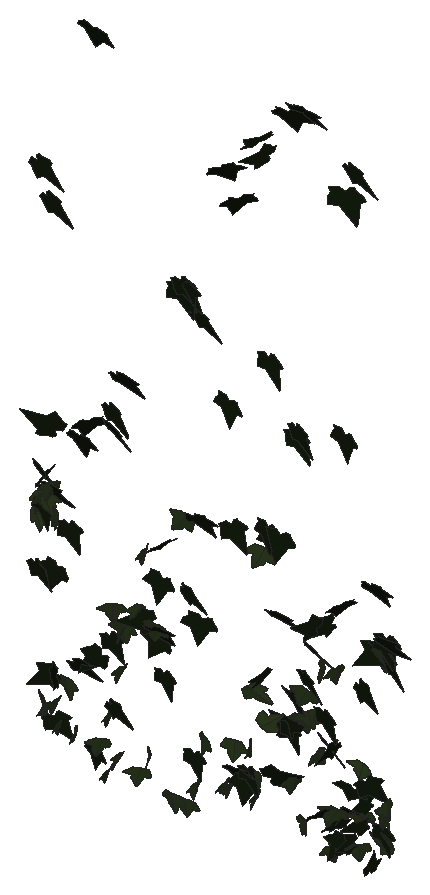
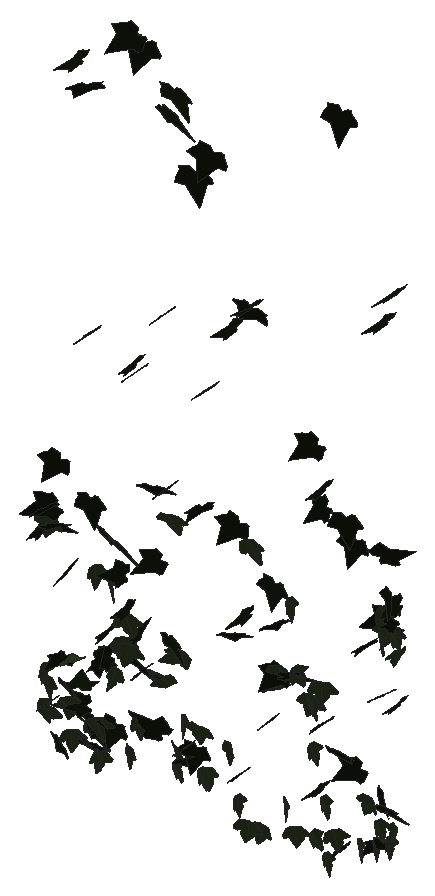
# SketchUp Ruby script. Lengths in inches.
U = 1.inch
M = Sketchup.active_model
def pt(a) = Geom::Point3d.new(a.map { |v| v * U })
def face(e, loops, mat)
  f = e.add_face(loops[0].map { |a| pt(a) })
  loops[1..].each { |l| e.add_face(l.map { |a| pt(a) }).erase! }
  f.material = f.back_material = mat if mat
  f
end
# faces: each face lists its corners as indices into pts; further lists are holes
def faces(e, pts, list, mat = nil) = list.each { |f| face(e, (f[0].is_a?(Array) ? f : [f]).map { |l| l.map { |i| pts[i] } }, mat) }
# xy, xz, yz: faces in a plane at the given z, y or x. An outline is a flat list of corners, or four numbers for a rectangle; further outlines are holes
def ring(l) = l.size == 4 ? [[l[0], l[1]], [l[2], l[1]], [l[2], l[3]], [l[0], l[3]]] : l.each_slice(2).to_a
def flat(e, list, mat, &to3) = list.each { |f| face(e, (f[0].is_a?(Array) ? f : [f]).map { |l| ring(l).map { |u, v| to3.(u, v) } }, mat) }
def xy(e, z, list, mat = nil) = flat(e, list, mat) { |x, y| [x, y, z] }
def xz(e, y, list, mat = nil) = flat(e, list, mat) { |x, z| [x, y, z] }
def yz(e, x, list, mat = nil) = flat(e, list, mat) { |y, z| [x, y, z] }
def lines(e, pts, list) = list.each { |a, b| e.add_line(pt(pts[a]), pt(pts[b])) }
# prism: a flat outline (further loops are holes) pulled along v
def prism(e, loops, v, mat = nil)
  f = face(e, loops, mat); d = Geom::Vector3d.new(v.map { |x| x * U })
  f.pushpull(f.normal.samedirection?(d) ? d.length : -d.length)
end
def box(e, o, s, mat = nil) = prism(e, [[o, [o[0] + s[0], o[1], o[2]], [o[0] + s[0], o[1] + s[1], o[2]], [o[0], o[1] + s[1], o[2]]]], [0, 0, s[2]], mat)
def at(x, y, z, deg = 0) = Geom::Transformation.translation(pt([x, y, z])) * Geom::Transformation.rotation(ORIGIN, Z_AXIS, deg.degrees)
def axes(o, x, y, z) = Geom::Transformation.new([*x, 0, *y, 0, *z, 0, *pt(o).to_a, 1])
def part(name) = M.definitions.add(name)
# library, detail: a bought-in or finely detailed component or shape, given as its bounding box
def library(name, o, s) = part(name).tap { |d| box(d.entities, o, s) }
def detail(e, o, s) = box(e.add_group.entities, o, s)
def put(e, d, t, mat = nil) = e.add_instance(d, t).tap { |i| i.material = mat if mat }
def group(e, t, mat = nil) = e.add_group.tap { |g| g.transformation = t; g.material = mat if mat }.entities
root = M.entities
M.materials.add("1026 AP 7946 SUNNY SIDE UP").color = [254, 231, 186]
M.materials.add("efeu1").color = [18, 25, 13]
M.materials.add("efeu2").color = [43, 57, 29]
c1 = part("ivyleaf_10")
p = [[0,0.5,-0.03],[-0.0625,2.02,-0.43],[-0.19,2.01,-0.46],[-0.54,1.05,-0.29],[-0.52,0.625,-0.18],[-0.83,0.76,-0.28],
  [-1.16,0.64,-0.33],[-1.15,0.33,-0.24],[-0.77,-0.39,0.02],[-0.3,-0.51,0.16],[0.04,-0.48,0.23],[-0.02,2.01,-0.4375],
  [-0.06,2.01,-0.43],[0.04,-0.49,0.23],[0.67,-0.49,0.14],[1.38,0.36,-0.2],[1.375,0.51,-0.24],[0.81,0.65,-0.19],
  [0.62,0.59,-0.15],[0.6,1.09,-0.28],[0.5,1.23,-0.31]]
faces(c1.entities,p,[[0,1,2,3,4,5,6,7,8,9,10],[11,12,0,13,14,15,16,17,18,19,20]],"efeu2")
c2 = part("ivyleaf_9")
p = [[1.54,2.16,1.25],[1.36,2.04,1.19],[-0.21,0.99,0.68],[-0.71,1.11,0.82],[-0.85,0.86,0.67],[-0.8,0.17,0.21],
  [-0.9,-0.01,0.1],[-0.67,-0.16,-0.02],[-0.08,-0.08,-0.05],[-0.03,-0.6,-0.4],[0.65,-0.88,-0.66],[0.83,-0.6,-0.49],
  [1.29,-0.42,-0.43],[1.8125,-0.07,-0.26],[1.21,0.44,0.15]]
faces(c2.entities,p,[[0,1,2,3,4,5,6,7,8,9,10,11,12,13,14]],"efeu1")
put(root,c1,axes([121.33,212.79,302.52],[0.10637,0.39079,-0.00968],[0.02001,-0.01398,-0.40837],[-0.61442,0.0672,-0.01498]),"1026 AP 7946 SUNNY SIDE UP")
put(root,c1,axes([121.55,212.8125,303.32],[0.06673,-0.37905,0.11263],[0.06236,-0.10747,-0.39263],[0.61813,0.05177,0.02745]),"1026 AP 7946 SUNNY SIDE UP")
put(root,c2,axes([121.34,212.72,299.95],[0.26024,-0.34424,-0.06742],[-0.02451,0.06291,-0.39289],[0.54987,0.16572,0.01439]),"1026 AP 7946 SUNNY SIDE UP")
put(root,c2,axes([121.39,212.77,304.82],[0.50632,-0.2219,-0.1012],[-0.11938,0.0607,-0.40245],[0.36159,0.33077,0.00883]),"1026 AP 7946 SUNNY SIDE UP")
put(root,c2,axes([122.21,212.83,306.92],[-0.05078,0.03558,0.41858],[-0.63945,0.02571,-0.03548],[-0.04487,-0.40658,0.03198]),"1026 AP 7946 SUNNY SIDE UP")
put(root,c1,axes([121.73,212.61,293.58],[-0.33327,0.29751,-0.06698],[0.04015,-0.06364,-0.37633],[-0.47774,-0.21289,0.0151]),"1026 AP 7946 SUNNY SIDE UP")
put(root,c2,axes([122.14,212.97,294.69],[-0.5677,0.0109,0.06133],[-0.0946,-0.02922,-0.37094],[-0.00938,-0.36474,0.0294]),"1026 AP 7946 SUNNY SIDE UP")
put(root,c1,axes([121.87,212.75,293.03],[0.00756,-0.36104,-0.03336],[0.0595,0.03067,-0.36972],[0.56658,0.0016,0.03927]),"1026 AP 7946 SUNNY SIDE UP")
put(root,c2,axes([121.65,212.84,303.01],[0.0399,-0.38612,0.09331],[0.00278,-0.09285,-0.39916],[0.62441,0.02508,-0.00419]),"1026 AP 7946 SUNNY SIDE UP")
put(root,c2,axes([121.55,212.65,319.99],[0.37125,-0.34932,-0.17132],[-0.0289,0.18222,-0.42522],[0.60632,0.22258,0.08463]),"1026 AP 7946 SUNNY SIDE UP")
put(root,c1,axes([121.85,212.78,303.5],[-0.54402,-0.18187,-0.0849],[0.20368,-0.0814,-0.38039],[0.23805,-0.34598,0.13143]),"1026 AP 7946 SUNNY SIDE UP")
put(root,c2,axes([122.06,212.32,304.62],[0.02868,0.31316,0.28228],[0.05693,0.27025,-0.32119],[-0.64997,0.03749,-0.01568]),"1026 AP 7946 SUNNY SIDE UP")
put(root,c1,axes([122.23,212.74,304.17],[-0.16107,-0.37373,0.10448],[0.00803,-0.10838,-0.39845],[0.60974,-0.0973,0.03285]),"1026 AP 7946 SUNNY SIDE UP")
put(root,c2,axes([121.84,212.72,303.97],[0.60813,-0.03029,0.10695],[0.15812,-0.04285,-0.39839],[0.06327,0.39819,-0.03237]),"1026 AP 7946 SUNNY SIDE UP")
put(root,c2,axes([122.63,212.46,294.99],[-0.04508,0.04129,-0.39829],[-0.58566,0.10915,0.04108],[0.17673,0.37224,0.03452]),"1026 AP 7946 SUNNY SIDE UP")
put(root,c2,axes([122.33,212.91,300.04],[-0.1812,-0.33573,0.14976],[-0.00027,-0.15433,-0.36347],[0.57646,-0.1056,0.0469]),"1026 AP 7946 SUNNY SIDE UP")
put(root,c1,axes([122.5,212.68,293.6],[0.01008,-0.37059,0.02268],[-0.00408,-0.02417,-0.38197],[0.58394,0.00623,-0.00306]),"1026 AP 7946 SUNNY SIDE UP")
put(root,c2,axes([122.11,212.67,318.38],[0.3947,-0.35863,-0.10135],[-0.00699,0.11337,-0.44606],[0.58386,0.2438,0.06317]),"1026 AP 7946 SUNNY SIDE UP")
put(root,c1,axes([122.54,212.55,302.875],[0.33528,-0.29784,-0.17526],[-0.06636,0.17406,-0.3711],[0.53392,0.20867,0.06394]),"1026 AP 7946 SUNNY SIDE UP")
put(root,c2,axes([122.45,212.66,292.78],[0.0045,-0.24534,-0.2768],[0.08535,0.26459,-0.24804],[0.56408,-0.03807,0.03974]),"1026 AP 7946 SUNNY SIDE UP")
put(root,c1,axes([122.73,212.61,292.625],[0.07917,-0.35089,-0.09058],[0.01544,0.08806,-0.364],[0.56784,0.04653,0.02252]),"1026 AP 7946 SUNNY SIDE UP")
put(root,c1,axes([122.96,212.82,294.67],[-0.51029,0.1557,-0.08413],[0.06055,-0.10614,-0.36284],[-0.2704,-0.3176,0.07751]),"1026 AP 7946 SUNNY SIDE UP")
put(root,c2,axes([123.02,212.92,302.34],[0.06958,-0.38131,-0.08499],[-0.00634,0.08039,-0.39495],[0.6127,0.04413,0.00557]),"1026 AP 7946 SUNNY SIDE UP")
put(root,c1,axes([123.51,212.72,292.36],[0.11564,-0.32495,-0.14498],[-0.04094,0.13649,-0.3424],[0.55415,0.07789,0.00496]),"1026 AP 7946 SUNNY SIDE UP")
put(root,c2,axes([123.71,212.74,307.09],[0.55846,0.04574,-0.20647],[-0.30488,-0.05996,-0.36794],[-0.10861,0.40351,-0.02883]),"1026 AP 7946 SUNNY SIDE UP")
put(root,c2,axes([123.67,212.6,295.91],[0.58034,0.04904,0.07753],[0.12618,-0.03962,-0.38048],[-0.06264,0.37453,-0.04815]),"1026 AP 7946 SUNNY SIDE UP")
put(root,c2,axes([124.23,212.75,308.01],[0.17855,0.37794,-0.12977],[-0.01863,-0.12995,-0.4065],[-0.62721,0.11145,-0.02487]),"1026 AP 7946 SUNNY SIDE UP")
put(root,c2,axes([124.71,212.91,296.55],[-0.58229,-0.02463,-0.05448],[0.0864,-0.03575,-0.38044],[0.03022,-0.37234,0.03792]),"1026 AP 7946 SUNNY SIDE UP")
put(root,c2,axes([124.625,212.59,327.68],[0.56003,0.08179,-0.31402],[-0.4724,-0.05518,-0.37664],[-0.15428,0.46584,0.01337]),"1026 AP 7946 SUNNY SIDE UP")
put(root,c2,axes([124.47,212.98,291.7],[-0.05063,-0.2928,0.19937],[0.03443,-0.19729,-0.30233],[0.55225,-0.01454,0.03713]),"1026 AP 7946 SUNNY SIDE UP")
put(root,c1,axes([124.875,212.79,292.35],[-0.32246,-0.28956,0.07943],[-0.02183,-0.08612,-0.36399],[0.47134,-0.20209,0.03748]),"1026 AP 7946 SUNNY SIDE UP")
put(root,c1,axes([125.28,212.78,291.06],[0.03805,-0.35139,-0.06364],[-0.01593,0.05921,-0.36245],[0.56023,0.02555,-0.00598]),"1026 AP 7946 SUNNY SIDE UP")
put(root,c1,axes([125.31,212.9,293.87],[0.06231,-0.35999,-0.01203],[0.00078,0.00975,-0.37304],[0.56626,0.0396,0.00184]),"1026 AP 7946 SUNNY SIDE UP")
put(root,c1,axes([125.6,212.74,299.31],[-0.43779,-0.25989,-0.00816],[0.02693,-0.00892,-0.39197],[0.40788,-0.27835,0.01713]),"1026 AP 7946 SUNNY SIDE UP")
put(root,c2,axes([125.38,212.85,297.67],[0.14543,-0.35271,-0.10857],[-0.01186,0.10477,-0.37455],[0.57782,0.09093,0.01964]),"1026 AP 7946 SUNNY SIDE UP")
put(root,c2,axes([125.36,212.77,308.22],[0.59667,-0.15909,-0.05563],[-0.09956,-0.01425,-0.42222],[0.24421,0.3829,-0.0362]),"1026 AP 7946 SUNNY SIDE UP")
put(root,c2,axes([125.42,212.77,309.07],[0.31942,-0.35968,-0.05875],[-0.0305,0.05218,-0.42516],[0.57133,0.20388,0.01015]),"1026 AP 7946 SUNNY SIDE UP")
put(root,c1,axes([125.85,212.9,291.97],[0.04888,-0.33321,0.11736],[-0.00514,-0.11653,-0.34517],[0.55466,0.02829,-0.01354]),"1026 AP 7946 SUNNY SIDE UP")
put(root,c2,axes([125.53,212.76,294.4],[0.3469,-0.27036,-0.13319],[-0.04821,0.13747,-0.35345],[0.46771,0.2147,0.06236]),"1026 AP 7946 SUNNY SIDE UP")
put(root,c1,axes([125.91,212.96,296.28],[-0.00159,-0.36779,0.0462],[0.00028,-0.04693,-0.37918],[0.58301,-0.00098,0.00031]),"1026 AP 7946 SUNNY SIDE UP")
put(root,c1,axes([126.08,212.875,298.38],[0.19251,-0.35677,0.04956],[0.00353,-0.0522,-0.3886],[0.56649,0.12157,-0.01442]),"1026 AP 7946 SUNNY SIDE UP")
put(root,c1,axes([126.09,212.77,298.52],[-0.59785,0.00285,-0.02962],[0.04436,-0.04652,-0.38908],[-0.00996,-0.37845,0.04535]),"1026 AP 7946 SUNNY SIDE UP")
put(root,c2,axes([126.04,212.6,310.95],[0.65732,0.0054,0.01686],[0.02629,-0.03378,-0.42947],[-0.00638,0.41699,-0.03255]),"1026 AP 7946 SUNNY SIDE UP")
put(root,c1,axes([126.9,212.86,299.625],[-0.08388,-0.3355,0.18576],[0.03107,-0.18617,-0.34826],[0.59953,-0.03729,0.04404]),"1026 AP 7946 SUNNY SIDE UP")
put(root,c1,axes([127.09,212.7,291.71],[-0.41796,-0.23407,0.05867],[-0.00568,-0.08285,-0.36026],[0.37925,-0.2592,0.05927]),"1026 AP 7946 SUNNY SIDE UP")
put(root,c2,axes([127.5,212.85,299.2],[-0.43002,-0.02854,0.27429],[-0.39245,-0.11133,-0.27688],[0.15324,-0.3652,0.06063]),"1026 AP 7946 SUNNY SIDE UP")
put(root,c1,axes([127.37,212.69,302.76],[0.06035,-0.39018,-0.04608],[0.03201,0.04464,-0.40285],[0.61632,0.03589,0.02543]),"1026 AP 7946 SUNNY SIDE UP")
put(root,c1,axes([127.76,212.51,292.8],[0.15864,-0.28812,-0.22136],[-0.05493,0.21257,-0.31167],[0.56094,0.1023,0.03209]),"1026 AP 7946 SUNNY SIDE UP")
put(root,c1,axes([128.01,212.66,299.21],[-0.5942,0.00973,0.06559],[-0.10117,-0.05282,-0.38579],[-0.00115,-0.37955,0.0531]),"1026 AP 7946 SUNNY SIDE UP")
put(root,c2,axes([128.01,212.96,298.45],[-0.29728,-0.28745,0.16028],[0.0311,-0.19119,-0.33675],[0.51424,-0.15461,0.11302]),"1026 AP 7946 SUNNY SIDE UP")
put(root,c2,axes([128.24,212.625,303.32],[0.14041,0.3847,0.09419],[0.00254,0.09115,-0.40587],[-0.62097,0.08736,0.01964]),"1026 AP 7946 SUNNY SIDE UP")
put(root,c2,axes([127.95,212.6,299.09],[0.57744,0.10817,-0.00508],[-0.00608,-0.00652,-0.3944],[-0.1702,0.36722,-0.00317]),"1026 AP 7946 SUNNY SIDE UP")
put(root,c2,axes([128.15,212.875,301.52],[-0.195,-0.36437,0.05171],[-0.01085,-0.05284,-0.39668],[0.57869,-0.12377,0.00999]),"1026 AP 7946 SUNNY SIDE UP")
put(root,c2,axes([128.25,212.97,296.79],[0.09727,-0.3651,0.02383],[-0.00158,-0.02573,-0.3816],[0.57545,0.06164,-0.00508]),"1026 AP 7946 SUNNY SIDE UP")
put(root,c1,axes([128.97,212.63,291.15],[-0.53807,0.10814,-0.01952],[0.00637,-0.05151,-0.36672],[-0.17268,-0.33886,0.04729]),"1026 AP 7946 SUNNY SIDE UP")
put(root,c1,axes([129.43,212.86,304.96],[-0.52621,0.04515,0.21978],[-0.34243,-0.07614,-0.33619],[0.00595,-0.38936,0.08883]),"1026 AP 7946 SUNNY SIDE UP")
put(root,c1,axes([129.66,212.71,291.08],[-0.56181,-0.03946,0.01615],[-0.01922,-0.03362,-0.36904],[0.06407,-0.35606,0.03093]),"1026 AP 7946 SUNNY SIDE UP")
put(root,c2,axes([129.3125,212.86,316.65],[0.25955,-0.39868,-0.07337],[0.04708,0.08631,-0.43972],[0.63445,0.15669,0.06265]),"1026 AP 7946 SUNNY SIDE UP")
put(root,c2,axes([129.45,212.72,316.5],[-0.3515,-0.13578,-0.36517],[0.51436,0.13802,-0.26676],[0.30055,-0.395,0.02945]),"1026 AP 7946 SUNNY SIDE UP")
put(root,c2,axes([129.55,212.79,301.5],[0.44393,-0.24145,-0.13668],[-0.09494,0.12916,-0.37765],[0.42161,0.28332,0.05888]),"1026 AP 7946 SUNNY SIDE UP")
put(root,c1,axes([130.19,212.71,292.13],[0.02128,-0.36446,-0.00022],[0.05924,-0.00044,-0.37372],[0.57002,0.01365,0.03885]),"1026 AP 7946 SUNNY SIDE UP")
put(root,c2,axes([130.02,212.8,293.5],[0.06534,-0.36411,0.00008],[-0.01063,-0.00293,-0.37748],[0.57243,0.04151,-0.00702]),"1026 AP 7946 SUNNY SIDE UP")
put(root,c2,axes([130.38,212.875,300.28],[-0.34237,-0.31015,-0.06145],[0.15513,-0.00012,-0.38161],[0.47122,-0.2253,0.08098]),"1026 AP 7946 SUNNY SIDE UP")
put(root,c1,axes([130.69,212.7,294.54],[-0.41987,0.25585,0.0646],[-0.17399,-0.03004,-0.36784],[-0.37529,-0.27231,0.09826]),"1026 AP 7946 SUNNY SIDE UP")
put(root,c2,axes([130.2,212.88,315.35],[0.41591,-0.33969,-0.05053],[0.01587,0.06719,-0.44025],[0.539,0.26013,0.05195]),"1026 AP 7946 SUNNY SIDE UP")
put(root,c2,axes([130.37,212.5,305.52],[0.62854,0.09278,-0.04282],[-0.05587,-0.03278,-0.42223],[-0.15014,0.4006,-0.02215]),"1026 AP 7946 SUNNY SIDE UP")
put(root,c2,axes([131.67,212.63,323.23],[0.41397,0.37438,0.02943],[0.05257,0.00878,-0.47089],[-0.5878,0.26445,-0.02139]),"1026 AP 7946 SUNNY SIDE UP")
put(root,c1,axes([131.89,212.58,292.84],[-0.02981,-0.34556,-0.10277],[0.0122,0.09752,-0.35595],[0.56456,-0.02035,0.00227]),"1026 AP 7946 SUNNY SIDE UP")
put(root,c1,axes([132.1,212.81,292.8125],[0.04357,-0.36183,0.02879],[-0.00078,-0.03013,-0.37401],[0.5709,0.02757,-0.00271]),"1026 AP 7946 SUNNY SIDE UP")
put(root,c2,axes([131.89,212.9,311.6],[-0.05636,-0.39316,0.14692],[0.02189,-0.14641,-0.40672],[0.65847,-0.02879,0.0261]),"1026 AP 7946 SUNNY SIDE UP")
put(root,c1,axes([132.3,212.71,294.89],[0.58598,-0.0019,0.03095],[0.04735,0.01769,-0.38338],[0.00074,0.37346,0.0205]),"1026 AP 7946 SUNNY SIDE UP")
put(root,c2,axes([132.56,212.7,321.99],[0.16832,0.42077,-0.14311],[-0.02245,-0.14201,-0.44763],[-0.69757,0.1061,-0.02012]),"1026 AP 7946 SUNNY SIDE UP")
put(root,c2,axes([132.26,212.63,305.73],[0.05843,-0.34975,-0.21873],[-0.02002,0.21011,-0.36101],[0.64142,0.03842,0.00866]),"1026 AP 7946 SUNNY SIDE UP")
put(root,c2,axes([132.54,212.58,293.76],[0.45318,0.16376,-0.16866],[-0.26686,-0.03058,-0.33757],[-0.24924,0.33052,0.05476]),"1026 AP 7946 SUNNY SIDE UP")
put(root,c2,axes([132.92,212.82,293.23],[-0.24103,-0.3314,-0.01154],[0.02338,0.00338,-0.37593],[0.52077,-0.15353,0.01154]),"1026 AP 7946 SUNNY SIDE UP")
put(root,c1,axes([133.13,212.76,295.06],[0.14966,-0.33413,-0.1452],[0.03356,0.1487,-0.35221],[0.56807,0.07924,0.05906]),"1026 AP 7946 SUNNY SIDE UP")
put(root,c2,axes([133,212.8125,293.76],[0.09877,-0.36001,-0.04218],[-0.00475,0.03896,-0.37624],[0.56936,0.06278,0.00418]),"1026 AP 7946 SUNNY SIDE UP")
put(root,c1,axes([133.46,212.85,292.6875],[0.11529,-0.34905,0.06272],[0.00406,-0.06366,-0.36766],[0.55767,0.07263,-0.01029]),"1026 AP 7946 SUNNY SIDE UP")
put(root,c1,axes([133.49,212.83,293.59],[0.39249,-0.26802,0.00356],[0.03774,0.01557,-0.3761],[0.41981,0.24918,0.03048]),"1026 AP 7946 SUNNY SIDE UP")
put(root,c2,axes([133.89,212.41,325.43],[-0.09156,0.45463,0.08265],[-0.17538,0.06206,-0.46014],[-0.70368,-0.07462,0.10393]),"1026 AP 7946 SUNNY SIDE UP")
put(root,c2,axes([134.04,212.81,324.59],[-0.46207,0.35597,0.01198],[-0.10815,-0.04452,-0.46835],[-0.54939,-0.29063,0.08212]),"1026 AP 7946 SUNNY SIDE UP")
put(root,c2,axes([133.91,212.71,298.71],[-0.22757,0.35634,0.04831],[-0.04335,0.03721,-0.39583],[-0.56307,-0.14688,0.01095]),"1026 AP 7946 SUNNY SIDE UP")
put(root,c1,axes([133.7,212.91,304.8125],[0.61004,0.00624,-0.09577],[-0.14541,-0.02405,-0.39923],[-0.01834,0.39823,-0.02028]),"1026 AP 7946 SUNNY SIDE UP")
put(root,c1,axes([133.4,212.6,298.03],[-0.36204,-0.08897,-0.30954],[0.48037,0.01644,-0.24651],[0.10617,-0.37778,0.05983]),"1026 AP 7946 SUNNY SIDE UP")
put(root,c2,axes([133.99,212.95,306.09],[0.00355,-0.39255,0.09228],[-0.01819,-0.09183,-0.40476],[0.63363,-0.00044,-0.01214]),"1026 AP 7946 SUNNY SIDE UP")
put(root,c2,axes([134.15,212.82,314.58],[0.11472,-0.42389,-0.01817],[-0.00195,0.01524,-0.44302],[0.66695,0.07296,0.00183]),"1026 AP 7946 SUNNY SIDE UP")
put(root,c1,axes([134.09,212.67,296.52],[0.39245,0.06289,-0.28919],[0.40586,0.11618,0.26359],[0.20095,-0.35748,0.03241]),"1026 AP 7946 SUNNY SIDE UP")
put(root,c2,axes([134.6875,212.86,305.96],[-0.41232,-0.27715,-0.13115],[0.24561,0.01987,-0.38062],[0.4107,-0.29013,0.09595]),"1026 AP 7946 SUNNY SIDE UP")
put(root,c2,axes([134.45,212.73,293.95],[0.045,-0.02351,0.4023],[0.57724,-0.13411,-0.03681],[0.21322,0.36802,0.01474]),"1026 AP 7946 SUNNY SIDE UP")
put(root,c2,axes([134.64,212.56,302.25],[0.61614,0.00004,0.0283],[0.04284,0.04919,-0.40021],[-0.00548,0.38971,0.05283]),"1026 AP 7946 SUNNY SIDE UP")
put(root,c2,axes([135.57,212.67,296.71],[-0.12822,0.20482,0.36225],[-0.4225,0.24071,-0.20792],[-0.47844,-0.26746,0.08653]),"1026 AP 7946 SUNNY SIDE UP")
put(root,c1,axes([135.53,212.85,294.16],[-0.15872,-0.35183,0.02045],[0.00144,-0.02299,-0.37714],[0.55429,-0.10069,0.00683]),"1026 AP 7946 SUNNY SIDE UP")
put(root,c2,axes([135.42,212.61,327.32],[0.59533,0.22012,-0.16183],[-0.20328,-0.09249,-0.45148],[-0.37478,0.39983,-0.01217]),"1026 AP 7946 SUNNY SIDE UP")
put(root,c2,axes([135.28,212.83,296.72],[0.12366,-0.3698,0.00899],[-0.00282,-0.01145,-0.38953],[0.58172,0.07856,-0.0038]),"1026 AP 7946 SUNNY SIDE UP")
put(root,c2,axes([135.84,212.76,298.07],[0.17285,-0.36529,0.07763],[-0.01832,0.07732,0.39328],[-0.58686,-0.11001,0.01059]),"1026 AP 7946 SUNNY SIDE UP")
put(root,c2,axes([135.6,212.86,311.28],[0.16473,-0.4031,-0.06475],[0.00465,0.06328,-0.42827],[0.64093,0.10315,0.01975]),"1026 AP 7946 SUNNY SIDE UP")
put(root,c2,axes([135.68,212.83,311.61],[0.28397,-0.37857,-0.03003],[-0.0211,0.02351,-0.43196],[0.5964,0.18108,-0.00098]),"1026 AP 7946 SUNNY SIDE UP")
put(root,c1,axes([136.09,212.82,297.5],[-0.56081,-0.12772,-0.04118],[0.0712,-0.01028,-0.3895],[0.19767,-0.35866,0.02346]),"1026 AP 7946 SUNNY SIDE UP")
put(root,c1,axes([136.33,212.71,298.82],[-0.55395,-0.06132,0.15511],[-0.20542,-0.10842,-0.36021],[0.15299,-0.36761,0.07797]),"1026 AP 7946 SUNNY SIDE UP")
put(root,c2,axes([135.81,212.7,327.64],[0.74158,0.02396,-0.00135],[-0.00576,0.04373,-0.48413],[-0.0373,0.46959,0.04793]),"1026 AP 7946 SUNNY SIDE UP")
put(root,c1,axes([136.21,212.59,292.4],[0.38251,-0.25225,-0.10752],[0.0108,0.14364,-0.34504],[0.42826,0.22168,0.10474]),"1026 AP 7946 SUNNY SIDE UP")
put(root,c2,axes([136.02,212.9375,299.48],[0.34955,-0.34275,0.0197],[-0.00966,-0.02906,-0.42048],[0.53987,0.2214,-0.02028]),"1026 AP 7946 SUNNY SIDE UP")
put(root,c1,axes([136.37,212.8,297.78],[-0.34302,-0.30459,-0.0775],[0.15105,0.02022,-0.37997],[0.46895,-0.22931,0.06571]),"1026 AP 7946 SUNNY SIDE UP")
put(root,c2,axes([136.85,212.59,302.26],[-0.38473,0.29657,0.12379],[-0.1661,0.0657,-0.39377],[-0.4739,-0.2638,0.03751]),"1026 AP 7946 SUNNY SIDE UP")
put(root,c2,axes([136.36,212.84,301.0625],[0.47602,-0.21752,0.12149],[0.15815,-0.06421,-0.38436],[0.35649,0.31895,0.00828]),"1026 AP 7946 SUNNY SIDE UP")
put(root,c1,axes([136.92,212.6875,295.99],[-0.10693,-0.30818,-0.24007],[0.12707,0.21823,-0.32277],[0.5924,-0.10244,0.0259]),"1026 AP 7946 SUNNY SIDE UP")
put(root,c2,axes([137.13,212.39,293.22],[0.20023,0.36361,0.12904],[0.05648,0.11794,-0.39618],[-0.60102,0.13222,0.00576]),"1026 AP 7946 SUNNY SIDE UP")
put(root,c1,axes([137.24,212.64,300.34],[0.23904,-0.32062,-0.19081],[-0.09829,0.17313,-0.36418],[0.57241,0.16362,0.01715]),"1026 AP 7946 SUNNY SIDE UP")
put(root,c2,axes([137.625,212.7,302.6875],[-0.5375,0.17718,-0.09901],[0.08598,-0.10261,-0.39174],[-0.30586,-0.34022,0.06388]),"1026 AP 7946 SUNNY SIDE UP")
put(root,c2,axes([137.15,212.875,297.99],[0.20692,-0.40159,0.03758],[-0.00057,-0.04089,-0.43539],[0.63439,0.13095,-0.01265]),"1026 AP 7946 SUNNY SIDE UP")
put(root,c2,axes([137.15,212.82,296.76],[0.56478,-0.21343,-0.05294],[-0.09031,0.00135,-0.42945],[0.33272,0.36267,-0.0267]),"1026 AP 7946 SUNNY SIDE UP")
put(root,c1,axes([137.79,212.93,293.33],[-0.51337,-0.16724,0.16133],[-0.18755,-0.1106,-0.37624],[0.30878,-0.34523,0.03969]),"1026 AP 7946 SUNNY SIDE UP")
put(root,c2,axes([137.65,213.02,296.54],[-0.2128,0.00789,-0.40579],[0.31845,-0.3559,-0.0811],[-0.53145,-0.21642,0.11388]),"1026 AP 7946 SUNNY SIDE UP")
put(root,c1,axes([137.75,212.6875,291.63],[-0.22636,-0.32246,-0.07247],[0.10227,0.04552,-0.36118],[0.50817,-0.1528,0.0404]),"1026 AP 7946 SUNNY SIDE UP")
put(root,c2,axes([137.99,212.86,293.06],[-0.29727,0.2868,-0.11401],[0.05932,-0.10921,-0.3534],[-0.48065,-0.19086,0.0269]),"1026 AP 7946 SUNNY SIDE UP")
put(root,c1,axes([137.89,212.63,291.75],[0.3185,-0.29674,-0.08058],[0.0035,0.09316,-0.36551],[0.48185,0.19546,0.05591]),"1026 AP 7946 SUNNY SIDE UP")
put(root,c1,axes([138.04,212.61,300.6],[-0.13946,-0.36774,-0.08035],[0.05125,0.07017,-0.38899],[0.5882,-0.0933,0.01484]),"1026 AP 7946 SUNNY SIDE UP")
put(root,c2,axes([138.28,212.36,293.01],[0.19031,0.25195,0.24162],[-0.11766,0.26059,-0.24862],[-0.52674,0.03282,0.14283]),"1026 AP 7946 SUNNY SIDE UP")
put(root,c2,axes([138.33,212.58,303.93],[0.07502,0.40071,-0.06024],[-0.0028,-0.06096,-0.41605],[-0.63727,0.04744,-0.00526]),"1026 AP 7946 SUNNY SIDE UP")
put(root,c2,axes([138.3,212.82,292.14],[-0.52877,-0.12234,-0.06534],[0.12362,-0.03514,-0.36381],[0.17735,-0.34027,0.05879]),"1026 AP 7946 SUNNY SIDE UP")
put(root,c2,axes([138.24,212.95,312.15],[-0.00931,-0.40484,0.12034],[0.02081,-0.11924,-0.41754],[0.66323,-0.00194,0.01479]),"1026 AP 7946 SUNNY SIDE UP")
put(root,c2,axes([138.85,212.69,292.28],[-0.49706,0.18241,-0.03321],[-0.00518,-0.07127,-0.37074],[-0.29151,-0.30977,0.06321]),"1026 AP 7946 SUNNY SIDE UP")
put(root,c2,axes([138.43,212.78,324.3],[-0.12705,-0.41301,-0.18712],[0.14058,0.16381,-0.4293],[0.69388,-0.10881,0.05271]),"1026 AP 7946 SUNNY SIDE UP")
put(root,c2,axes([138.71,212.92,294.81],[-0.31463,-0.27509,0.18355],[0.26558,-0.26661,-0.22822],[0.44321,-0.03552,0.26706]),"1026 AP 7946 SUNNY SIDE UP")
put(root,c2,axes([138.65,212.9,325.52],[0.45208,-0.356,-0.06078],[0.02188,0.08378,-0.46644],[0.56648,0.28087,0.06652]),"1026 AP 7946 SUNNY SIDE UP")
put(root,c2,axes([138.61,212.66,293.8125],[0.49543,-0.10195,0.16131],[0.27184,0.03981,-0.33022],[0.11344,0.34984,0.08684]),"1026 AP 7946 SUNNY SIDE UP")
put(root,c1,axes([139.26,212.76,292.2],[-0.35023,-0.28755,0.00482],[0.02292,-0.01926,-0.37405],[0.45167,-0.22199,0.02272]),"1026 AP 7946 SUNNY SIDE UP")
put(root,c1,axes([139.3,212.8,293.8],[-0.48666,-0.19597,0.00288],[0.01274,-0.02009,-0.37686],[0.30794,-0.30887,0.02014]),"1026 AP 7946 SUNNY SIDE UP")
put(root,c2,axes([139.5625,212.66,293.49],[-0.48205,0.20099,0.02378],[-0.05304,-0.01155,-0.3766],[-0.31346,-0.30714,0.02715]),"1026 AP 7946 SUNNY SIDE UP")
put(root,c1,axes([139.1,213.09,295.94],[-0.44999,-0.122,0.23911],[0.27402,-0.34571,0.03204],[0.30936,0.12876,0.31943]),"1026 AP 7946 SUNNY SIDE UP")
put(root,c2,axes([139.72,212.74,294.53],[-0.48889,0.18639,-0.05854],[0.04775,-0.06134,-0.37191],[-0.30316,-0.31026,0.03582]),"1026 AP 7946 SUNNY SIDE UP")
put(root,c2,axes([139.4,212.61,300.25],[0.33717,-0.29861,-0.19525],[-0.17007,0.15357,-0.37782],[0.52798,0.24016,0.00298]),"1026 AP 7946 SUNNY SIDE UP")
put(root,c2,axes([139.92,212.61,291.36],[0.14284,0.13314,0.33647],[-0.03377,0.338,-0.13413],[-0.55246,0.01377,0.0952]),"1026 AP 7946 SUNNY SIDE UP")
put(root,c2,axes([140.32,212.93,302.11],[-0.51782,-0.15943,0.17177],[-0.19215,-0.12776,-0.37321],[0.30888,-0.34675,0.0558]),"1026 AP 7946 SUNNY SIDE UP")
put(root,c2,axes([139.84,212.51,295.72],[0.0334,-0.19949,-0.33839],[0.02835,0.328,-0.2028],[0.6021,-0.00438,0.02832]),"1026 AP 7946 SUNNY SIDE UP")
put(root,c2,axes([139.97,212.69,305.37],[0.61418,0.06062,-0.09316],[-0.13885,-0.02279,-0.40724],[-0.1009,0.40036,-0.00667]),"1026 AP 7946 SUNNY SIDE UP")
put(root,c1,axes([140.875,212.64,292.89],[-0.03904,0.02336,-0.41424],[-0.5368,0.21281,0.03569],[0.33647,0.34223,0.00887]),"1026 AP 7946 SUNNY SIDE UP")
put(root,c1,axes([140.5625,212.67,302.24],[-0.62435,0.06422,-0.01303],[0.00607,-0.05686,-0.41074],[-0.10285,-0.39319,0.05486]),"1026 AP 7946 SUNNY SIDE UP")
put(root,c1,axes([140.67,212.59,294.32],[0.44914,-0.2089,-0.122],[-0.04286,0.15292,-0.34823],[0.37423,0.26824,0.10654]),"1026 AP 7946 SUNNY SIDE UP")
put(root,c2,axes([140.45,212.82,293.37],[0.06247,-0.36358,0.00822],[0.0087,-0.0095,-0.37681],[0.57184,0.03986,0.00483]),"1026 AP 7946 SUNNY SIDE UP")
put(root,c2,axes([140.59,212.89,302.85],[-0.0038,-0.40277,-0.06419],[-0.00859,0.06005,-0.41454],[0.64025,-0.00159,-0.00594]),"1026 AP 7946 SUNNY SIDE UP")
put(root,c2,axes([140.46,212.5,302.86],[0.58274,0.05803,0.15862],[0.24615,-0.01013,-0.38513],[-0.07811,0.40106,-0.03028]),"1026 AP 7946 SUNNY SIDE UP")
put(root,c1,axes([140.8125,212.64,294.875],[-0.00692,-0.36978,-0.03746],[0.15548,0.03186,-0.36714],[0.56285,-0.01335,0.10096]),"1026 AP 7946 SUNNY SIDE UP")
put(root,c2,axes([140.75,212.81,301.84],[0.37789,-0.32154,-0.04948],[-0.09294,0.01323,-0.4115],[0.50226,0.24437,-0.03892]),"1026 AP 7946 SUNNY SIDE UP")
